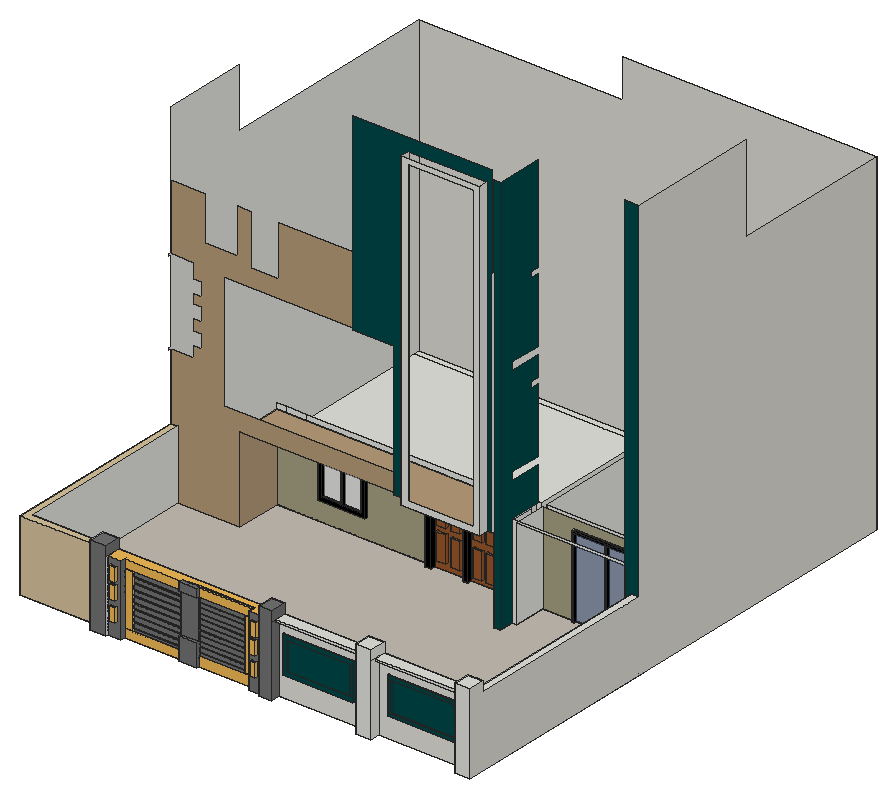
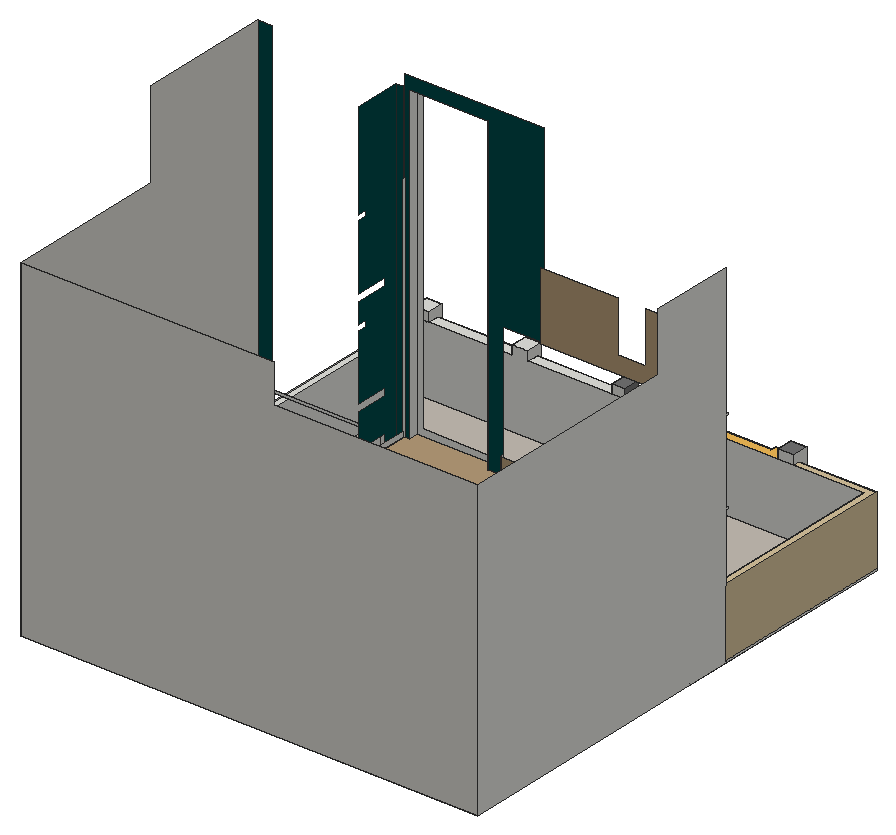
# SketchUp Ruby script. Lengths in inches.
U = 1.inch
M = Sketchup.active_model
def pt(a) = Geom::Point3d.new(a.map { |v| v * U })
def face(e, loops, mat)
  f = e.add_face(loops[0].map { |a| pt(a) })
  loops[1..].each { |l| e.add_face(l.map { |a| pt(a) }).erase! }
  f.material = f.back_material = mat if mat
  f
end
# faces: each face lists its corners as indices into pts; further lists are holes
def faces(e, pts, list, mat = nil) = list.each { |f| face(e, (f[0].is_a?(Array) ? f : [f]).map { |l| l.map { |i| pts[i] } }, mat) }
# xy, xz, yz: faces in a plane at the given z, y or x. An outline is a flat list of corners, or four numbers for a rectangle; further outlines are holes
def ring(l) = l.size == 4 ? [[l[0], l[1]], [l[2], l[1]], [l[2], l[3]], [l[0], l[3]]] : l.each_slice(2).to_a
def flat(e, list, mat, &to3) = list.each { |f| face(e, (f[0].is_a?(Array) ? f : [f]).map { |l| ring(l).map { |u, v| to3.(u, v) } }, mat) }
def xy(e, z, list, mat = nil) = flat(e, list, mat) { |x, y| [x, y, z] }
def xz(e, y, list, mat = nil) = flat(e, list, mat) { |x, z| [x, y, z] }
def yz(e, x, list, mat = nil) = flat(e, list, mat) { |y, z| [x, y, z] }
def lines(e, pts, list) = list.each { |a, b| e.add_line(pt(pts[a]), pt(pts[b])) }
# prism: a flat outline (further loops are holes) pulled along v
def prism(e, loops, v, mat = nil)
  f = face(e, loops, mat); d = Geom::Vector3d.new(v.map { |x| x * U })
  f.pushpull(f.normal.samedirection?(d) ? d.length : -d.length)
end
def box(e, o, s, mat = nil) = prism(e, [[o, [o[0] + s[0], o[1], o[2]], [o[0] + s[0], o[1] + s[1], o[2]], [o[0], o[1] + s[1], o[2]]]], [0, 0, s[2]], mat)
def at(x, y, z, deg = 0) = Geom::Transformation.translation(pt([x, y, z])) * Geom::Transformation.rotation(ORIGIN, Z_AXIS, deg.degrees)
def axes(o, x, y, z) = Geom::Transformation.new([*x, 0, *y, 0, *z, 0, *pt(o).to_a, 1])
def part(name) = M.definitions.add(name)
# library, detail: a bought-in or finely detailed component or shape, given as its bounding box
def library(name, o, s) = part(name).tap { |d| box(d.entities, o, s) }
def detail(e, o, s) = box(e.add_group.entities, o, s)
def put(e, d, t, mat = nil) = e.add_instance(d, t).tap { |i| i.material = mat if mat }
def group(e, t, mat = nil) = e.add_group.tap { |g| g.transformation = t; g.material = mat if mat }.entities
root = M.entities
M.materials.add("[0034_Wheat]").color = [214, 194, 156]
M.materials.add("[0035_Tan]").color = [181, 155, 120]
M.materials.add("[0079_Teal]").color = [0, 71, 71]
M.materials.add("[0137_Black]").color = [0, 0, 0]
M.materials.add("[Color M05]").color = [114, 114, 114]
M.materials.add("[Field Rectangle Tile]").color = [196, 189, 179]
M.materials.add("[Marble Carrara Gold Floor Tile]").color = [225, 223, 217]
M.materials.add("[Stone Coursed Rough]").color = [165, 160, 130]
M.materials.add("[Terrazzo Tile Light]").color = [219, 217, 210]
M.materials.add("[Terrazzo]").color = [241, 186, 86]
M.materials.add("[Translucent Glass Blue]").color = [52, 78, 124]
M.materials["[Translucent Glass Blue]"].alpha = 0.5
M.materials.add("[Translucent Glass Gray]").color = [201, 201, 201]
M.materials["[Translucent Glass Gray]"].alpha = 0.5
M.materials.add("[Wood Cherry Original]").color = [152, 86, 42]
xy(root,0,[[446.99,0,446.99,12,322.26,12,322.26,3,307.87,3,307.87,12,6.1875,12,6.1875,313.125,290.9375,313.125,290.9375,307.125,298.48,307.125,298.48,313.125,339.22,313.125,339.22,307.125,345.22,307.125,345.22,313.125,379.96,313.125,379.96,307.125,387.5,307.125,387.5,313.125,423.03,313.125,423.03,252.8125,431.125,252.8125,431.125,271.56,437.125,271.56,437.125,313.125,477.12,313.125,477.12,310.125,480.12,310.125,480.12,313.125,519.5,313.125,519.5,310.125,522.23,310.125,522.23,313.125,556.18,313.125,556.18,310.125,559.18,310.125,559.18,313.125,577.1875,313.125,577.1875,0,574.85,0,574.85,12,467.27,12,467.27,0],[105.5,0,125.95,12],[322.26,0,339.09,12],[577.1875,0,594.5625,270.3125],[125.95,3,143.04,12],
  [[423.03,252.8125,423.03,319.125,431.125,319.125,431.125,643.9375,6.1875,643.9375,6.1875,652.9375,594.5625,652.9375,594.5625,313.125,437.125,313.125,437.125,271.56,431.125,271.56,431.125,252.8125],[437.125,319.125,568.1875,643.9375]],[577.1875,270.3125,594.5625,313.125],[290.9375,307.125,298.48,307.125,298.48,313.125,339.22,313.125,339.22,307.125,345.22,307.125,345.22,313.125,379.96,313.125,379.96,307.125,387.5,307.125,387.5,313.125,423.03,313.125,423.03,319.125,106.1875,319.125,106.1875,313.125,290.9375,313.125],[477.12,310.125,480.12,313.125],[519.5,310.125,522.23,313.125],
  [556.18,310.125,559.18,313.125],[6.1875,313.125,106.1875,319.125],[6.1875,319.125,431.125,643.9375],[437.125,319.125,568.1875,643.9375]])
xy(root,0,[[215.47,6,215.47,9,216.92,9,216.92,12,226.19,12,226.19,6],[226.19,6,238.07,12],[215.47,9,216.92,12]],"[Color M05]")
xy(root,0,[[143.04,9,215.47,12],[238.07,9,307.87,12]],"[Terrazzo]")
xy(root,3,[[15.1875,21,585.5625,21,585.5625,270.3125,577.1875,270.3125,577.1875,313.125,559.18,313.125,559.18,310.125,556.18,310.125,556.18,313.125,522.23,313.125,522.23,310.125,519.5,310.125,519.5,313.125,480.12,313.125,480.12,310.125,477.12,310.125,477.12,313.125,437.125,313.125,437.125,271.56,431.125,271.56,431.125,252.8125,423.03,252.8125,423.03,313.125,387.5,313.125,387.5,307.125,379.96,307.125,379.96,313.125,345.22,313.125,345.22,307.125,339.22,307.125,339.22,313.125,298.48,313.125,298.48,307.125,290.9375,307.125,290.9375,313.125,95.27,313.125,95.27,253.5,15.1875,253.5]],"[Field Rectangle Tile]")
xy(root,9.35,[[366.08,310.125,378.02,313.125]])
xy(root,9.66,[[349.7,310.125,361.64,313.125]])
xy(root,10.72,[[143.04,9,153.77,10.875],[215.47,9,216.92,12],[153.77,10,215.47,12],[143.04,10.875,153.77,12]])
xy(root,10.72,[[153.77,9,215.47,10]],"[Terrazzo]")
xy(root,11.5,[[143.04,10.875,153.77,12]])
xy(root,11.5,[[143.04,9,153.77,10.875]],"[Terrazzo]")
xy(root,11.6,[[321.33,310.125,333.27,313.125]])
xy(root,12.04,[[238.07,10,297.68,12]])
xy(root,12.04,[[238.07,9,307.87,9,307.87,12,297.68,12,297.68,10,238.07,10]],"[Terrazzo]")
xy(root,12.6,[[302.77,310.125,314.7,313.125]])
xy(root,12.94,[[153.77,10,215.47,12]])
xy(root,13.63,[[297.68,9,307.87,12]],"[Terrazzo]")
xy(root,14.85,[[153.77,10,215.47,12]],"[Color M05]")
xy(root,15.36,[[238.07,10,297.68,12]],"[Color M05]")
xy(root,16.62,[[238.07,10,297.68,12]],"[Color M05]")
xy(root,18.75,[[129.89,0,137.27,3],[310.71,0,318.08,3]],"[Terrazzo]")
xy(root,20.38,[[153.77,10,215.47,12]],"[Color M05]")
xy(root,21.8,[[238.07,10,297.68,12]],"[Color M05]")
xy(root,22.29,[[153.77,10,215.47,12]],"[Color M05]")
xy(root,23.05,[[238.07,10,297.68,12]],"[Color M05]")
xy(root,27.43,[[345.52,10,435.96,12],[480.27,10,570.71,12]],"[0079_Teal]")
xy(root,27.82,[[153.77,10,215.47,12]],"[Color M05]")
xy(root,28.24,[[238.07,10,297.68,12]],"[Color M05]")
xy(root,28.71,[[149.99,310.125,211.11,313.125]])
xy(root,28.98,[[215.47,9,226.19,12],[226.19,9,238.07,12]])
xy(root,28.98,[[215.47,6,238.07,9]],"[Color M05]")
xy(root,29.49,[[238.07,10,297.68,12]],"[Color M05]")
xy(root,29.73,[[153.77,12,215.47,12.6875]])
xy(root,29.73,[[153.77,10,215.47,12]],"[Color M05]")
xy(root,31.96,[[484.81,10,566.18,12]],"[0079_Teal]")
xy(root,32.32,[[350.41,10,431.07,12]],"[0079_Teal]")
xy(root,33.85,[[155.13,310.125,179.85,313.125],[182.85,310.125,205.97,313.125]],"[0137_Black]")
xy(root,34.67,[[238.07,10,297.68,12]],"[Color M05]")
xy(root,35.26,[[153.77,12,215.47,12.6875]])
xy(root,35.26,[[153.77,10,215.47,12]],"[Color M05]")
xy(root,35.93,[[238.07,10,297.68,12]],"[Color M05]")
xy(root,35.94,[[129.89,0,137.27,3],[310.71,0,318.08,3]],"[Terrazzo]")
xy(root,37.17,[[153.77,10,215.47,12]],"[Color M05]")
xy(root,41.11,[[238.07,10,297.68,12]],"[Color M05]")
xy(root,42.37,[[238.07,10,297.68,12]],"[Color M05]")
xy(root,42.69,[[153.77,10,215.47,12]],"[Color M05]")
xy(root,42.97,[[366.08,310.125,378.02,313.125]],"[Wood Cherry Original]")
xy(root,43.29,[[349.7,310.125,361.64,313.125]],"[Wood Cherry Original]")
xy(root,44.13,[[129.89,0,137.27,3],[310.33,0,317.71,3]],"[Terrazzo]")
xy(root,44.6,[[153.77,10,215.47,12]],"[Color M05]")
xy(root,45.22,[[321.33,310.125,333.27,313.125]],"[Wood Cherry Original]")
xy(root,46.22,[[302.77,310.125,314.7,313.125]],"[Wood Cherry Original]")
xy(root,47.55,[[238.07,10,297.68,12]],"[Color M05]")
xy(root,48.8,[[238.07,10,297.68,12]],"[Color M05]")
xy(root,50.13,[[153.77,10,215.47,12]],"[Color M05]")
xy(root,52.04,[[153.77,10,215.47,12]],"[Color M05]")
xy(root,53.85,[[302.77,310.125,314.7,313.125],[321.33,310.125,333.27,313.125],[349.7,310.125,361.64,313.125],[366.08,310.125,378.02,313.125]],"[Wood Cherry Original]")
xy(root,53.99,[[238.07,10,297.68,12]],"[Color M05]")
xy(root,55.24,[[238.07,10,297.68,12]],"[Color M05]")
xy(root,57.57,[[153.77,10,215.47,12]],"[Color M05]")
xy(root,59.48,[[153.77,10,215.47,12]],"[Color M05]")
xy(root,60.42,[[238.07,10,297.68,12]],"[Color M05]")
xy(root,61.32,[[129.89,0,137.27,3],[310.33,0,317.71,3]],"[Terrazzo]")
xy(root,61.68,[[238.07,10,297.68,12]],"[Color M05]")
xy(root,65.01,[[153.77,10,215.47,12]],"[Color M05]")
xy(root,65.38,[[311.08,0,318.46,3]])
xy(root,65.38,[[129.89,0,137.27,3]],"[Terrazzo]")
xy(root,66.86,[[238.07,10,297.68,12]],"[Color M05]")
xy(root,66.92,[[153.77,11.5,215.47,12]])
xy(root,66.92,[[153.77,10,215.47,11.5]],"[Color M05]")
xy(root,68.12,[[238.07,10,297.68,12]],"[Color M05]")
xy(root,70.16,[[350.41,10,431.07,12]],"[0079_Teal]")
xy(root,70.52,[[484.81,10,566.18,12]],"[0079_Teal]")
xy(root,72.44,[[153.77,11.5,215.47,12]])
xy(root,72.44,[[153.77,10,215.47,11.5]],"[Color M05]")
xy(root,73.3,[[238.07,10,297.68,12]],"[Color M05]")
xy(root,73.85,[[153.77,10,215.47,12]],"[Color M05]")
xy(root,74.55,[[238.07,10,297.68,12]],"[Color M05]")
xy(root,75.05,[[345.52,10,435.96,12],[480.27,10,570.71,12]],"[0079_Teal]")
xy(root,79.38,[[153.77,10,215.47,12],[143.04,10.875,153.77,12]])
xy(root,79.38,[[143.04,9,153.77,10.875],[297.68,9,307.87,12]],"[Terrazzo]")
xy(root,79.74,[[238.07,10,297.68,12]])
xy(root,80.4,[[215.47,9,238.07,12],[143.04,10.875,153.77,12]])
xy(root,80.4,[[215.47,6,238.07,9]],"[Color M05]")
xy(root,80.4,[[143.04,9,153.77,10.875],[153.77,9,215.47,12],[238.07,9,307.87,12]],"[Terrazzo]")
xy(root,82.57,[[129.89,0,137.27,3],[311.08,0,318.46,3]],"[Terrazzo]")
xy(root,87.47,[[302.77,310.125,314.7,313.125],[321.33,310.125,333.27,313.125],[349.7,310.125,361.64,313.125],[366.08,310.125,378.02,313.125]],"[Wood Cherry Original]")
xy(root,88.15,[[467.27,6,574.85,12]])
xy(root,88.28,[[339.13,6,446.99,12]])
xy(root,91.125,[[125.91,0,125.95,12],[339.09,0,339.13,12],[467.24,0,467.27,0,467.27,6,574.85,6,574.85,21,467.24,21],[339.13,6,446.99,21],[574.85,21,585.5625,21.01],
  [585.5625,21.01,594.5625,270.3125]])
xy(root,91.125,[[6.1875,12,105.5,12,105.5,21,15.1875,21,15.1875,253.5,6.1875,253.5]],"[0034_Wheat]")
xy(root,91.125,[[215.47,6,226.19,12],[226.19,6,238.07,12]],"[Color M05]")
xy(root,91.125,[[125.95,3,143.04,3,143.04,9,215.47,9,215.47,12,307.87,12,307.87,3,322.26,3,322.26,21,125.91,21,125.91,12,125.95,12],[238.07,9,307.87,12]],"[Terrazzo]")
xy(root,96.02,[[298.48,307.125,339.22,313.125],[345.22,307.125,379.96,313.125]],"[0137_Black]")
xy(root,98.375,[[155.13,310.125,179.85,313.125],[182.85,310.125,205.97,313.125]],"[0137_Black]")
xy(root,103.125,[[446.99,0,467.24,21],[574.85,0,594.5625,0,594.5625,21.01,585.5625,21.01,585.5625,21,574.85,21]])
xy(root,103.125,[[105.5,0,125.91,21],[322.26,0,339.13,21]],"[Color M05]")
xy(root,103.52,[[149.99,310.125,211.11,313.125]],"[0137_Black]")
xy(root,103.5625,[[290.9375,307.125,387.5,313.125]],"[0137_Black]")
xy(root,105.5625,[[480.12,310.125,519.5,313.125],[522.49,310.125,556.18,313.125]])
xy(root,108.5625,[[477.12,310.125,559.18,313.125]],"[0137_Black]")
xy(root,113.0625,[[315.58,237.8125,315.58,249.8125,296.54,249.8125,296.54,253.5,95.27,253.5,95.27,313.125,423.03,313.125,423.03,249.8125,416.24,249.8125,416.24,237.8125]],"[0035_Tan]")
xz(root,0,[[446.99,0,467.27,0,467.27,91.125,467.24,91.125,467.24,103.125,446.99,103.125],[574.85,0,594.5625,103.125]])
xz(root,0,[[105.5,0,125.95,0,125.95,91.125,125.91,91.125,125.91,103.125,105.5,103.125],[322.26,0,339.09,0,339.09,91.125,339.13,91.125,339.13,103.125,322.26,103.125]],"[Color M05]")
xz(root,0,[[129.89,18.75,137.27,35.94],[310.71,18.75,318.08,35.94],[129.89,44.13,137.27,61.32],[310.33,44.13,317.71,61.32],[129.89,65.38,137.27,82.57],
  [311.08,65.38,318.46,82.57]],"[Terrazzo]")
xz(root,3,[[[125.95,0,143.04,91.125],[129.89,65.38,137.27,82.57],[129.89,44.13,137.27,61.32],[129.89,18.75,137.27,35.94]],[[307.87,0,322.26,91.125],[310.71,18.75,318.08,35.94],[310.33,44.13,317.71,61.32],[311.08,65.38,318.46,82.57]]],"[Color M05]")
xz(root,6,[[467.27,88.15,574.85,91.125],[339.13,88.28,446.99,91.125]])
xz(root,6,[[215.47,0,238.07,28.98],[215.47,80.4,238.07,91.125]],"[Color M05]")
xz(root,9,[[215.47,28.98,238.07,80.4]],"[Color M05]")
xz(root,9,[[143.04,0,216.92,10.72],[238.07,0,307.87,12.04],[143.04,11.5,153.77,79.38],[297.68,13.63,307.87,79.38],[143.04,80.4,215.47,91.125],
  [238.07,80.4,307.87,91.125]],"[Terrazzo]")
xz(root,10,[[[345.52,27.43,435.96,75.05],[350.41,32.32,431.07,70.16]],[[480.27,27.43,570.71,75.05],[484.81,31.96,566.18,70.52]]],"[0079_Teal]")
xz(root,10,[[153.77,10.72,215.47,12.94],[238.07,12.04,297.68,15.36],[153.77,14.85,215.47,20.38],[238.07,16.62,297.68,21.8],[153.77,22.29,215.47,27.82],
  [238.07,23.05,297.68,28.24],[238.07,29.49,297.68,34.67],[153.77,29.73,215.47,35.26],[238.07,35.93,297.68,41.11],[153.77,37.17,215.47,42.69],
  [238.07,42.37,297.68,47.55],[153.77,44.6,215.47,50.13],[238.07,48.8,297.68,53.99],[153.77,52.04,215.47,57.57],[238.07,55.24,297.68,60.42],
  [153.77,59.48,215.47,65.01],[238.07,61.68,297.68,66.86],[153.77,66.92,215.47,72.44],[238.07,68.12,297.68,73.3],[153.77,73.85,215.47,79.38],
  [238.07,74.55,297.68,79.74]],"[Color M05]")
xz(root,10.875,[[143.04,10.72,153.77,11.5],[143.04,79.38,153.77,80.4]])
xz(root,11.5,[[153.77,66.92,215.47,72.44]])
xz(root,12,[[143.04,0,143.04,10.72,153.77,10.72,153.77,7.42,215.47,7.42,215.47,0],[215.47,0,216.92,7.42],[216.92,0,216.92,10.72,215.47,10.72,215.47,28.98,226.19,28.98,226.19,0],[226.19,0,238.07,28.98],[238.07,0,297.68,2.49],
  [297.68,0,297.68,2.49,238.07,2.49,238.07,3.74,297.68,3.74,297.68,8.92,238.07,8.92,238.07,10.18,297.68,10.18,297.68,12.04,307.87,12.04,307.87,0],[238.07,3.74,297.68,8.92],[153.77,7.42,215.47,10.72],[215.47,7.42,216.92,10.72],[238.07,10.18,297.68,12.04],
  [143.04,10.72,153.77,11.5],[153.77,10.72,215.47,12.94],[143.04,11.5,153.77,79.38],[297.68,12.04,307.87,13.63],[153.77,12.94,215.47,14.85],
  [297.68,13.63,307.87,79.38],[153.77,14.85,215.47,20.38],[238.07,15.36,297.68,16.62],[153.77,20.38,215.47,22.29],[238.07,21.8,297.68,23.05],
  [153.77,22.29,215.47,27.82],[153.77,27.82,215.47,29.73],[238.07,28.24,297.68,29.49],[215.47,28.98,226.19,80.4],[226.19,28.98,238.07,80.4],
  [153.77,29.73,215.47,35.26],[238.07,34.67,297.68,35.93],[153.77,35.26,215.47,37.17],[153.77,37.17,215.47,42.69],[238.07,41.11,297.68,42.37],
  [153.77,42.69,215.47,44.6],[153.77,44.6,215.47,50.13],[238.07,47.55,297.68,48.8],[153.77,50.13,215.47,52.04],[153.77,52.04,215.47,57.57],
  [238.07,53.99,297.68,55.24],[153.77,57.57,215.47,59.48],[153.77,59.48,215.47,65.01],[238.07,60.42,297.68,61.68],[153.77,65.01,215.47,66.92],
  [238.07,66.86,297.68,68.12],[153.77,72.44,215.47,73.85],[238.07,73.3,297.68,74.55],[143.04,79.38,153.77,80.4],[153.77,79.38,215.47,80.4],
  [297.68,79.38,307.87,79.38,307.87,80.4,238.07,80.4,238.07,79.74,297.68,79.74],[215.47,80.4,215.47,91.125,226.19,91.125,226.19,80.59,238.07,80.59,238.07,80.4],[238.07,80.4,307.87,91.125],[226.19,80.59,238.07,91.125]])
xz(root,12,[[6.1875,0,105.5,91.125]],"[0034_Wheat]")
xz(root,12,[[484.81,31.96,566.18,70.52],[350.41,32.32,431.07,70.16]],"[0079_Teal]")
xz(root,12,[[[339.09,0,446.99,0,446.99,88.28,339.13,88.28,339.13,91.125,339.09,91.125],[345.52,27.43,435.96,75.05]],[[467.27,0,574.85,88.15],[480.27,27.43,570.71,75.05]]],"[Marble Carrara Gold Floor Tile]")
xz(root,12.6875,[[153.77,29.73,215.47,35.26]])
xz(root,21,[[15.1875,3,15.1875,91.125,446.99,91.125,446.99,103.125,467.24,103.125,467.24,91.125,585.5625,91.125,585.5625,3],[105.5,91.125,125.91,103.125],[322.26,91.125,339.13,103.125],[574.85,91.125,585.5625,103.125]])
xz(root,21.01,[[585.5625,91.125,594.5625,103.125]])
xz(root,237.8125,[[[315.58,113.0625,416.24,514.78],[323.96,121,409.46,509.47]]])
xz(root,249.8125,[[296.54,113.0625,315.58,113.0625,315.58,514.78,416.24,514.78,416.24,113.0625,423.03,113.0625,423.03,531.37,243.98,531.37,243.98,284.3125,296.54,284.3125]],"[0079_Teal]")
xz(root,252.8125,[[423.03,0,431.125,3]])
xz(root,252.8125,[[423.03,3,431.125,518.125]],"[0079_Teal]")
xz(root,253.5,[[6.1875,3,15.1875,91.125]])
xz(root,253.5,[[15.1875,3,95.27,3,95.27,113.0625,296.54,113.0625,296.54,136.125,74.71,136.125,74.71,284.3125,243.98,284.3125,243.98,371.77,145.3125,371.77,145.3125,306.52,109.1875,306.52,109.1875,371.77,92.36,371.77,92.36,314.76,50.28,314.76,50.28,371.77,6.1875,371.77,6.1875,287.35,36.19,287.35,36.19,268.61,46.11,268.61,46.11,251.74,36.19,251.74,36.19,239.3,46.11,239.3,46.11,222.43,36.19,222.43,36.19,208.43,46.11,208.43,46.11,191.55,36.19,191.55,36.19,177.18,6.1875,177.18,6.1875,91.125,15.1875,91.125]],"[0035_Tan]")
xz(root,270.3125,[[577.1875,3,585.5625,3,585.5625,91.125,594.5625,91.125,594.5625,541.5625,577.1875,541.5625]],"[0079_Teal]")
xz(root,271.56,[[431.125,0,437.125,3],[431.125,3,437.125,3,437.125,120,577.1875,120,577.1875,123,431.125,123]])
xz(root,307.125,[[290.9375,0,298.48,3],[339.22,0,345.22,3],[379.96,0,387.5,3]])
xz(root,307.125,[[290.9375,3,298.48,3,298.48,96.02,339.22,96.02,339.22,3,345.22,3,345.22,96.02,379.96,96.02,379.96,3,387.5,3,387.5,103.5625,290.9375,103.5625]],"[0137_Black]")
xz(root,310.125,[[477.12,0,480.12,3],[519.5,0,522.23,3],[556.18,0,559.18,3]])
xz(root,310.125,[[522.23,0,522.49,105.5625,556.18,105.5625,556.18,3,559.18,3,559.18,108.5625,477.12,108.5625,477.12,3,480.12,3,480.12,105.5625,519.5,105.5625,519.5,3,522.23,3],[[149.99,28.71,211.11,103.52],[155.13,33.85,179.85,98.375],[182.85,33.85,205.97,98.375]]],"[0137_Black]")
xz(root,310.125,[[366.08,9.35,378.02,42.97],[349.7,9.66,361.64,43.29],[321.33,11.6,333.27,45.22],[302.77,12.6,314.7,46.22],[302.77,53.85,314.7,87.47],
  [321.33,53.85,333.27,87.47],[349.7,53.85,361.64,87.47],[366.08,53.85,378.02,87.47]],"[Wood Cherry Original]")
xz(root,313.125,[[95.27,0,97.1875,3],[97.1875,0,106.1875,3],[106.1875,0,290.9375,3],[298.48,0,339.22,3],[345.22,0,379.96,3],
  [387.5,0,423.03,3],[437.125,0,477.12,3],[477.12,0,477.12,108.5625,559.18,108.5625,559.18,0,556.18,0,556.18,105.5625,522.49,105.5625,522.24,3,522.23,3,522.23,0,519.5,0,519.5,105.5625,480.12,105.5625,480.12,0],[480.12,0,519.5,3],[522.23,0,522.23,3,522.24,3],
  [522.23,0,522.24,3,522.24,0],[522.24,0,556.18,3],[559.18,0,568.1875,3],[568.1875,0,577.1875,3],[568.1875,3,577.1875,120],
  [95.27,113.0625,106.1875,120],[106.1875,113.0625,133.46,120],[133.46,113.0625,423.03,120]])
xz(root,313.125,[[[95.27,3,290.9375,3,290.9375,103.5625,387.5,103.5625,387.5,3,423.03,3,423.03,113.0625,95.27,113.0625],[149.99,28.71,211.11,103.52]],[437.125,3,477.12,3,477.12,108.5625,559.18,108.5625,559.18,3,568.1875,3,568.1875,120,437.125,120]],"[Stone Coursed Rough]")
xz(root,313.125,[[480.12,3,519.5,105.5625],[522.24,3,556.18,3,556.18,105.5625,522.49,105.5625]],"[Translucent Glass Blue]")
xz(root,313.125,[[155.13,33.85,179.85,98.375],[182.85,33.85,205.97,98.375]],"[Translucent Glass Gray]")
xz(root,313.125,[[[298.48,3,339.22,96.02],[302.77,53.85,314.7,87.47],[321.33,53.85,333.27,87.47],[321.33,11.6,333.27,45.22],[302.77,12.6,314.7,46.22]],[[345.22,3,379.96,96.02],[349.7,53.85,361.64,87.47],[366.08,53.85,378.02,87.47],[366.08,9.35,378.02,42.97],[349.7,9.66,361.64,43.29]]],"[Wood Cherry Original]")
xz(root,319.125,[[423.03,0,431.125,120],[437.125,0,568.1875,120]])
xz(root,643.9375,[[437.125,0,568.1875,120]])
xz(root,652.9375,[[6.1875,0,6.1875,380.6875,269.04,380.6875,269.04,430.25,594.5625,430.25,594.5625,0]],"[Terrazzo Tile Light]")
yz(root,6.1875,[[12,0,253.5,3],[253.5,0,253.5,177.18,251.5,177.18,251.5,178.93,253.5,178.93,253.5,285.5,251.5,285.5,251.5,287.35,253.5,287.35,253.5,456,363.1875,456,363.1875,380.6875,652.9375,380.6875,652.9375,0]])
yz(root,6.1875,[[12,3,253.5,91.125]],"[0034_Wheat]")
yz(root,15.1875,[[21,3,253.5,91.125]])
yz(root,95.27,[[253.5,3,313.125,113.0625]],"[0035_Tan]")
yz(root,105.5,[[0,0,0,103.125,21,103.125,21,91.125,12,91.125,12,0]])
yz(root,125.91,[[0,91.125,21,103.125]],"[Color M05]")
yz(root,125.95,[[0,0,3,91.125],[3,0,12,91.125]])
yz(root,129.89,[[0,18.75,3,35.94],[0,44.13,3,61.32],[0,65.38,3,82.57]],"[Terrazzo]")
yz(root,137.27,[[0,18.75,3,35.94],[0,44.13,3,61.32],[0,65.38,3,82.57]],"[Terrazzo]")
yz(root,143.04,[[9,0,12,10.72],[10.875,10.72,12,11.5],[9,11.5,12,79.38],[10.875,79.38,12,80.4]])
yz(root,143.04,[[3,0,9,0,9,10.72,10.875,10.72,10.875,11.5,9,11.5,9,79.38,10.875,79.38,10.875,80.4,9,80.4,9,91.125,3,91.125]],"[Color M05]")
yz(root,149.99,[[310.125,28.71,313.125,103.52]])
yz(root,153.77,[[10,10.72,10.875,11.5],[10.875,10.72,12,11.5],[10,11.5,12,12.94],[10,14.85,12,20.38],[10,22.29,12,27.82],
  [10,29.73,12,35.26],[12,29.73,12.6875,35.26],[10,37.17,12,42.69],[10,44.6,12,50.13],[10,52.04,12,57.57],
  [10,59.48,12,65.01],[10,66.92,11.5,72.44],[11.5,66.92,12,72.44],[10,73.85,12,79.38],[10.875,79.38,12,80.4]])
yz(root,153.77,[[9,11.5,10,11.5,10,12.94,12,12.94,12,14.85,10,14.85,10,20.38,12,20.38,12,22.29,10,22.29,10,27.82,12,27.82,12,29.73,10,29.73,10,35.26,12,35.26,12,37.17,10,37.17,10,42.69,12,42.69,12,44.6,10,44.6,10,50.13,12,50.13,12,52.04,10,52.04,10,57.57,12,57.57,12,59.48,10,59.48,10,65.01,12,65.01,12,66.92,10,66.92,10,72.44,12,72.44,12,73.85,10,73.85,10,79.38,9,79.38]],"[Terrazzo]")
yz(root,155.13,[[310.125,33.85,313.125,98.375]],"[0137_Black]")
yz(root,179.85,[[310.125,33.85,313.125,98.375]])
yz(root,182.85,[[310.125,33.85,313.125,98.375]],"[0137_Black]")
yz(root,205.97,[[310.125,33.85,313.125,98.375]])
yz(root,211.11,[[310.125,28.71,313.125,103.52]],"[0137_Black]")
yz(root,215.47,[[10,10.72,12,12.94],[10,14.85,12,20.38],[10,22.29,12,27.82],[10,29.73,12,35.26],[12,29.73,12.6875,35.26],
  [10,37.17,12,42.69],[10,44.6,12,50.13],[10,52.04,12,57.57],[10,59.48,12,65.01],[10,66.92,11.5,72.44],
  [11.5,66.92,12,72.44],[10,73.85,12,79.38]])
yz(root,215.47,[[6,0,12,10.72],[6,10.72,6,28.98,12,28.98,12,27.82,10,27.82,10,22.29,12,22.29,12,20.38,10,20.38,10,14.85,12,14.85,12,12.94,10,12.94,10,10.72],[9,28.98,9,80.4,12,80.4,12,79.38,10,79.38,10,73.85,12,73.85,12,72.44,10,72.44,10,66.92,12,66.92,12,65.01,10,65.01,10,59.48,12,59.48,12,57.57,10,57.57,10,52.04,12,52.04,12,50.13,10,50.13,10,44.6,12,44.6,12,42.69,10,42.69,10,37.17,12,37.17,12,35.26,10,35.26,10,29.73,12,29.73,12,28.98],[6,80.4,9,91.125]],"[Color M05]")
yz(root,216.92,[[9,0,12,10.72]])
yz(root,238.07,[[9,0,12,12.04],[10,12.04,12,15.36],[10,16.62,12,21.8],[10,23.05,12,28.24],[10,29.49,12,34.67],
  [10,35.93,12,41.11],[10,42.37,12,47.55],[10,48.8,12,53.99],[10,55.24,12,60.42],[10,61.68,12,66.86],
  [10,68.12,12,73.3],[10,74.55,12,79.74],[9,80.4,12,80.59],[9,80.59,12,91.125]])
yz(root,238.07,[[6,0,9,0,9,12.04,10,12.04,10,15.36,12,15.36,12,16.62,10,16.62,10,21.8,12,21.8,12,23.05,10,23.05,10,28.24,12,28.24,12,28.98,6,28.98],[9,28.98,12,28.98,12,29.49,10,29.49,10,34.67,12,34.67,12,35.93,10,35.93,10,41.11,12,41.11,12,42.37,10,42.37,10,47.55,12,47.55,12,48.8,10,48.8,10,53.99,12,53.99,12,55.24,10,55.24,10,60.42,12,60.42,12,61.68,10,61.68,10,66.86,12,66.86,12,68.12,10,68.12,10,73.3,12,73.3,12,74.55,10,74.55,10,79.74,12,79.74,12,80.4,9,80.4],[6,80.59,9,91.125]],"[Color M05]")
yz(root,290.9375,[[307.125,0,313.125,3]])
yz(root,290.9375,[[307.125,3,313.125,103.5625]],"[0137_Black]")
yz(root,296.54,[[249.8125,113.0625,253.5,136.125]])
yz(root,297.68,[[10,12.04,12,13.63],[10,13.63,12,15],[10,15,12,15.36],[10,16.62,12,21.44],[10,21.44,12,21.8],
  [10,23.05,12,27.88],[10,27.88,12,28.24],[10,29.49,12,34.32],[10,34.32,12,34.67],[10,35.93,12,40.75],
  [10,40.75,12,41.11],[10,42.37,12,47.19],[10,47.19,12,47.55],[10,48.8,12,53.63],[10,53.63,12,53.99],
  [10,55.24,12,60.07],[10,60.07,12,60.42],[10,61.68,12,66.5],[10,66.5,12,66.86],[10,68.12,12,72.94],
  [10,72.94,12,73.3],[10,74.55,12,79.38],[10,79.38,12,79.74]])
yz(root,297.68,[[9,13.63,9,79.38,10,79.38,10,74.55,12,74.55,12,73.3,10,73.3,10,68.12,12,68.12,12,66.86,10,66.86,10,61.68,12,61.68,12,60.42,10,60.42,10,55.24,12,55.24,12,53.99,10,53.99,10,48.8,12,48.8,12,47.55,10,47.55,10,42.37,12,42.37,12,41.11,10,41.11,10,35.93,12,35.93,12,34.67,10,34.67,10,29.49,12,29.49,12,28.24,10,28.24,10,23.05,12,23.05,12,21.8,10,21.8,10,16.62,12,16.62,12,15.36,10,15.36,10,13.63]],"[Terrazzo]")
yz(root,298.48,[[307.125,0,313.125,3]])
yz(root,298.48,[[307.125,3,313.125,96.02]],"[0137_Black]")
yz(root,302.77,[[310.125,12.6,313.125,46.22],[310.125,53.85,313.125,87.47]],"[Wood Cherry Original]")
yz(root,307.87,[[9,0,12,12.04],[9,13.63,12,79.38],[9,80.4,12,91.125]])
yz(root,307.87,[[3,0,3,91.125,9,91.125,9,80.4,12,80.4,12,79.38,9,79.38,9,13.63,12,13.63,12,12.04,9,12.04,9,0]],"[Color M05]")
yz(root,310.33,[[0,44.13,3,61.32]],"[Terrazzo]")
yz(root,310.71,[[0,18.75,3,35.94]])
yz(root,311.08,[[0,65.38,3,82.57]],"[Terrazzo]")
yz(root,314.7,[[310.125,12.6,313.125,46.22],[310.125,53.85,313.125,87.47]],"[Wood Cherry Original]")
yz(root,315.58,[[237.8125,113.0625,249.8125,514.78]])
yz(root,317.71,[[0,44.13,3,61.32]],"[Terrazzo]")
yz(root,318.08,[[0,18.75,3,35.94]],"[Terrazzo]")
yz(root,318.46,[[0,65.38,3,82.57]],"[Terrazzo]")
yz(root,321.33,[[310.125,11.6,313.125,45.22],[310.125,53.85,313.125,87.47]],"[Wood Cherry Original]")
yz(root,322.26,[[3,0,12,91.125]])
yz(root,322.26,[[0,0,0,103.125,21,103.125,21,91.125,3,91.125,3,0]],"[Color M05]")
yz(root,333.27,[[310.125,11.6,313.125,45.22],[310.125,53.85,313.125,87.47]],"[Wood Cherry Original]")
yz(root,339.09,[[0,0,12,91.125]],"[Color M05]")
yz(root,339.13,[[6,88.28,12,91.125]])
yz(root,339.13,[[0,91.125,21,103.125]],"[Color M05]")
yz(root,339.22,[[307.125,0,313.125,3]])
yz(root,339.22,[[307.125,3,313.125,96.02]],"[0137_Black]")
yz(root,345.22,[[307.125,0,313.125,3]])
yz(root,345.22,[[307.125,3,313.125,96.02]],"[0137_Black]")
yz(root,345.52,[[10,27.43,12,75.05]],"[0079_Teal]")
yz(root,349.7,[[310.125,9.66,313.125,43.29],[310.125,53.85,313.125,87.47]],"[Wood Cherry Original]")
yz(root,350.41,[[10,32.32,12,70.16]],"[0079_Teal]")
yz(root,361.64,[[310.125,9.66,313.125,43.29],[310.125,53.85,313.125,87.47]],"[Wood Cherry Original]")
yz(root,366.08,[[310.125,9.35,313.125,42.97],[310.125,53.85,313.125,87.47]],"[Wood Cherry Original]")
yz(root,378.02,[[310.125,9.35,313.125,42.97],[310.125,53.85,313.125,87.47]],"[Wood Cherry Original]")
yz(root,379.96,[[307.125,0,313.125,3]])
yz(root,379.96,[[307.125,3,313.125,96.02]],"[0137_Black]")
yz(root,387.5,[[307.125,0,313.125,3]])
yz(root,387.5,[[307.125,3,313.125,103.5625]],"[0137_Black]")
yz(root,416.24,[[237.8125,113.0625,249.8125,514.78]])
yz(root,423.03,[[252.8125,0,313.125,3],[313.125,0,319.125,120],[252.8125,3,313.125,113.0625],[249.8125,113.0625,252.8125,411],[252.8125,113.0625,313.125,120]])
yz(root,431.07,[[10,32.32,12,70.16]],"[0079_Teal]")
yz(root,431.125,[[252.8125,0,271.56,3],[319.125,0,643.9375,120]])
yz(root,431.125,[[252.8125,3,271.56,3,271.56,123,313.125,123,313.125,166.28,271.56,166.28,271.56,176.29,313.125,176.29,313.125,259.41,301.125,259.41,301.125,267,313.125,267,313.125,293.48,271.56,293.48,271.56,303.01,313.125,303.01,313.125,387,301.125,387,301.125,394.0625,313.125,394.0625,313.125,518.125,252.8125,518.125]],"[0079_Teal]")
yz(root,435.96,[[10,27.43,12,75.05]],"[0079_Teal]")
yz(root,437.125,[[271.56,0,313.125,3],[319.125,0,643.9375,120],[271.56,3,313.125,120]])
yz(root,446.99,[[0,0,0,103.125,21,103.125,21,91.125,6,91.125,6,88.28,12,88.28,12,0],[6,88.28,12,91.125]])
yz(root,467.24,[[0,91.125,21,103.125]])
yz(root,467.27,[[0,0,12,0,12,88.15,6,88.15,6,91.125,0,91.125],[6,88.15,12,91.125]])
yz(root,477.12,[[310.125,0,313.125,3],[310.125,3,313.125,108.5625]])
yz(root,480.12,[[310.125,0,313.125,3]])
yz(root,480.12,[[310.125,3,313.125,105.5625]],"[0137_Black]")
yz(root,480.27,[[10,27.43,12,75.05]],"[0079_Teal]")
yz(root,484.81,[[10,31.96,12,70.52]],"[0079_Teal]")
yz(root,519.5,[[310.125,0,313.125,3]])
yz(root,519.5,[[310.125,3,313.125,105.5625]],"[0137_Black]")
yz(root,522.23,[[310.125,0,313.125,3]])
yz(root,556.18,[[310.125,0,313.125,3]])
yz(root,556.18,[[310.125,3,313.125,105.5625]],"[0137_Black]")
yz(root,559.18,[[310.125,0,313.125,3]])
yz(root,559.18,[[310.125,3,313.125,108.5625]],"[0137_Black]")
yz(root,566.18,[[10,31.96,12,70.52]],"[0079_Teal]")
yz(root,568.1875,[[319.125,0,643.9375,120]])
yz(root,570.71,[[10,27.43,12,75.05]],"[0079_Teal]")
yz(root,574.85,[[0,0,0,103.125,21,103.125,21,91.125,6,91.125,6,88.15,12,88.15,12,0],[6,88.15,12,91.125]])
yz(root,577.1875,[[270.3125,0,313.125,3],[270.3125,3,313.125,120]])
yz(root,585.5625,[[21,3,270.3125,91.125],[21,91.125,21.01,103.125]])
yz(root,594.5625,[[0,0,652.9375,0,652.9375,430.25,443.1875,430.25,443.1875,541.5625,270.3125,541.5625,270.3125,91.125,21.01,91.125,21.01,103.125,0,103.125]],"[Terrazzo Tile Light]")
p = [[522.23,313.125,0],[522.24,313.125,3],[522.49,313.125,105.5625],[522.49,310.125,105.5625],[522.23,310.125,0],[95.27,313.125,3],
  [6.1875,313.125,3],[568.1875,304.125,3],[568.18,304.125,3],[585.5625,270.3125,3],[594.5625,270.3125,3],[143.04,12,91.125],
  [143.04,12,80.4]]
faces(root,p,[[0,1,2,3,4]],"[0137_Black]")
lines(root,p,[[5,6],[7,8],[9,10],[11,12]])
